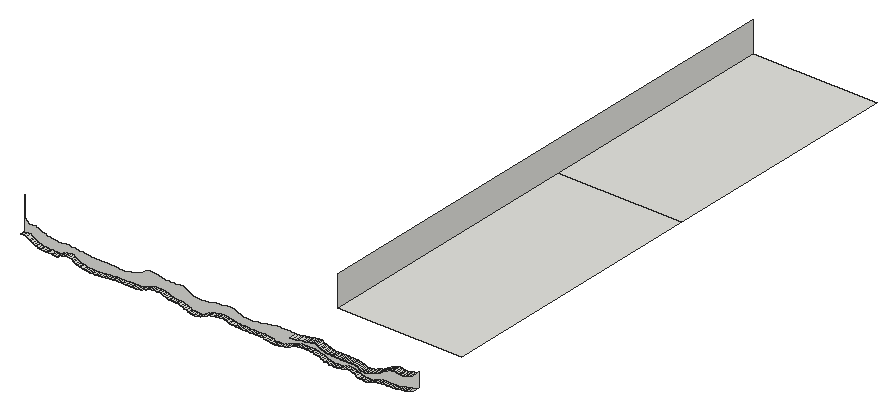
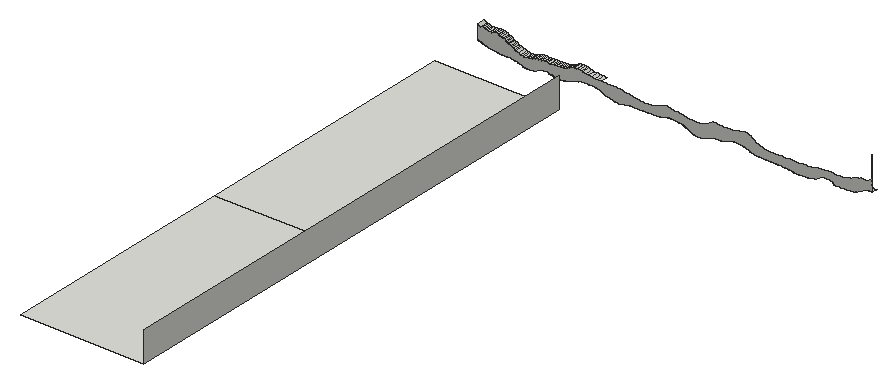
# SketchUp Ruby script. Lengths in inches.
U = 1.inch
M = Sketchup.active_model
def pt(a) = Geom::Point3d.new(a.map { |v| v * U })
def face(e, loops, mat)
  f = e.add_face(loops[0].map { |a| pt(a) })
  loops[1..].each { |l| e.add_face(l.map { |a| pt(a) }).erase! }
  f.material = f.back_material = mat if mat
  f
end
# faces: each face lists its corners as indices into pts; further lists are holes
def faces(e, pts, list, mat = nil) = list.each { |f| face(e, (f[0].is_a?(Array) ? f : [f]).map { |l| l.map { |i| pts[i] } }, mat) }
# xy, xz, yz: faces in a plane at the given z, y or x. An outline is a flat list of corners, or four numbers for a rectangle; further outlines are holes
def ring(l) = l.size == 4 ? [[l[0], l[1]], [l[2], l[1]], [l[2], l[3]], [l[0], l[3]]] : l.each_slice(2).to_a
def flat(e, list, mat, &to3) = list.each { |f| face(e, (f[0].is_a?(Array) ? f : [f]).map { |l| ring(l).map { |u, v| to3.(u, v) } }, mat) }
def xy(e, z, list, mat = nil) = flat(e, list, mat) { |x, y| [x, y, z] }
def xz(e, y, list, mat = nil) = flat(e, list, mat) { |x, z| [x, y, z] }
def yz(e, x, list, mat = nil) = flat(e, list, mat) { |y, z| [x, y, z] }
def lines(e, pts, list) = list.each { |a, b| e.add_line(pt(pts[a]), pt(pts[b])) }
# prism: a flat outline (further loops are holes) pulled along v
def prism(e, loops, v, mat = nil)
  f = face(e, loops, mat); d = Geom::Vector3d.new(v.map { |x| x * U })
  f.pushpull(f.normal.samedirection?(d) ? d.length : -d.length)
end
def box(e, o, s, mat = nil) = prism(e, [[o, [o[0] + s[0], o[1], o[2]], [o[0] + s[0], o[1] + s[1], o[2]], [o[0], o[1] + s[1], o[2]]]], [0, 0, s[2]], mat)
def at(x, y, z, deg = 0) = Geom::Transformation.translation(pt([x, y, z])) * Geom::Transformation.rotation(ORIGIN, Z_AXIS, deg.degrees)
def axes(o, x, y, z) = Geom::Transformation.new([*x, 0, *y, 0, *z, 0, *pt(o).to_a, 1])
def part(name) = M.definitions.add(name)
# library, detail: a bought-in or finely detailed component or shape, given as its bounding box
def library(name, o, s) = part(name).tap { |d| box(d.entities, o, s) }
def detail(e, o, s) = box(e.add_group.entities, o, s)
def put(e, d, t, mat = nil) = e.add_instance(d, t).tap { |i| i.material = mat if mat }
def group(e, t, mat = nil) = e.add_group.tap { |g| g.transformation = t; g.material = mat if mat }.entities
root = M.entities
xy(root,237.65,[[2039.58,2402.3,2040.27,2404.3],[2040.27,2402.3,2040.89,2404.3]])
xy(root,238.18,[[2133.53,2402.3,2134.21,2404.3]])
xy(root,238.33,[[2048.68,2402.3,2049.23,2404.3],[2049.23,2402.3,2049.91,2404.3]])
xy(root,238.34,[[2050.59,2402.3,2051.52,2404.3],[2051.52,2402.3,2052.01,2404.3],[2052.01,2402.3,2052.77,2404.3],[2052.77,2402.3,2053.4,2404.3],[2053.4,2402.3,2054.15,2404.3],
  [2054.15,2402.3,2054.77,2404.3],[2054.77,2402.3,2055.54,2404.3],[2055.54,2402.3,2056.16,2404.3]])
xy(root,238.62,[[2100.06,2402.3,2100.83,2404.3],[2100.83,2402.3,2101.46,2404.3],[2101.46,2402.3,2102.22,2404.3],[2102.22,2402.3,2102.84,2404.3],[2102.84,2402.3,2103.69,2404.3],
  [2103.69,2402.3,2104.33,2404.3],[2104.33,2402.3,2104.95,2404.3]])
xy(root,238.625,[[2098.64,2402.3,2099.5,2404.3]])
xy(root,238.89,[[2154.45,2402.3,2155.13,2404.3]])
xy(root,238.9,[[2155.89,2402.3,2156.51,2404.3],[2156.51,2402.3,2157.28,2404.3]])
xy(root,240.43,[[2122.73,2402.3,2123.3,2404.3]])
xy(root,241.52,[[2010.28,2402.3,2010.34,2404.3]])
xy(root,242.28,[[2140.55,2401.37,2141.0625,2404.3]])
xy(root,242.3,[[2138.79,2401.37,2139.46,2404.3]])
xy(root,242.33,[[2136.38,2401.37,2136.96,2404.3]])
xy(root,242.625,[[2115.89,2425.46,2164.35,2532.83],[2115.89,2532.83,2164.35,2628.15]])
xz(root,2404.3,[[2079.2,236.98,2078.59,237.01,2077.9,237.04,2077.14,237.11,2076.45,237.2,2075.92,237.33,2075.25,237.68,2074.3125,237.96,2073.75,238.28,2072.97,238.43,2072.19,238.78,2071.52,238.79,2070.98,238.8,2070.22,238.83,2069.47,238.875,2068.9,238.94,2068.32,239.04,2067.66,239.29,2067.08,239.53,2066.55,239.7,2065.86,239.92,2065.23,240.11,2064.45,240.27,2063.83,240.25,2063.125,240.23,2062.36,240.19,2061.6875,240.12,2061.03,240.03,2060.39,239.85,2059.84,239.52,2059.28,239.35,2058.69,239.18,2058.18,238.86,2057.49,238.72,2056.67,238.59,2056.16,238.34,2050.59,238.34,2049.91,238.33,2048.68,238.33,2047.96,238.32,2047.11,238.3,2046.48,238.28,2045.73,238.26,2045.1,238.15,2044.34,238.13,2043.79,238.1,2042.9375,237.98,2042.32,237.94,2041.56,237.89,2040.89,237.65,2039.58,237.65,2038.89,237.66,2038.14,237.67,2037.54,237.68,2036.93,237.71,2036.22,237.76,2035.53,237.82,2034.87,237.9,2033.93,238.21,2033.46,238.31,2032.55,238.43,2031.9,238.74,2031.32,239.11,2030.74,239.38,2030.28,239.71,2029.58,240.11,2028.89,240.09,2028.23,240.05,2027.64,239.99,2026.91,239.88,2026.36,239.69,2025.78,239.55,2025.22,238.9375,2024.69,238.77,2023.95,238.79,2023.08,238.8,2022.57,238.82,2021.53,238.92,2020.84,238.93,2020.14,238.94,2019.44,238.97,2018.76,239.03,2018.07,239.09,2017.29,239.19,2016.78,239.52,2016.22,239.64,2015.77,239.86,2014.98,240.2,2014.38,240.59,2013.84,240.85,2012.82,241.55,2011.55,241.69,2010.34,241.52,2010.34,246.2,2011.91,244.96,2013.3,244.9375,2014.55,244.92,2014.77,244.61,2015.33,244.54,2016.09,244.41,2016.76,244.11,2017.28,243.95,2017.94,243.79,2018.46,243.48,2019.1,243.3,2019.6875,243.14,2020.17,243.06,2020.89,242.85,2021.47,242.78,2022.28,242.73,2022.82,242.68,2023.49,242.51,2024.01,242.46,2024.55,242.58,2025.18,242.57,2025.81,242.81,2026.38,242.86,2026.94,242.89,2027.58,242.92,2028.01,242.625,2028.62,242.65,2029.17,242.62,2029.8,242.58,2030.36,242.57,2031,242.48,2031.66,242.38,2032.32,242.34,2032.99,242.24,2034.16,241.96,2034.93,241.89,2035.75,241.83,2036.35,241.78,2037.12,241.75,2037.57,241.74,2038.12,241.72,2039.38,241.7,2040.11,241.69,2040.78,241.68,2041.37,241.68,2041.86,241.67,2042.5625,241.74,2043.13,241.75,2045.13,241.75,2045.62,241.67,2046.15,241.66,2046.76,241.57,2047.3,241.53,2047.92,241.51,2048.47,241.49,2049.17,241.48,2049.83,241.47,2050.4,241.46,2051.11,241.6,2051.84,241.85,2052.51,241.91,2053.41,242.1,2054.18,242.46,2054.88,242.78,2055.65,242.97,2056.18,243.23,2056.58,243.48,2057.1,243.72,2057.4375,244.12,2057.91,244.39,2058.39,244.73,2058.875,244.87,2059.46,244.95,2060.14,245.01,2060.79,244.81,2061.36,244.7,2061.84,244.67,2062.45,244.55,2062.99,244.51,2063.45,244.25,2064.2,244.11,2064.76,244.04,2065.38,243.99,2066.1,243.95,2066.6,243.93,2067.29,243.91,2067.86,243.89,2068.56,243.88,2069.21,243.94,2069.85,243.95,2070.41,244.1,2071.04,244.13,2071.52,244.15,2072.04,244.17,2072.56,244.18,2073.16,243.8,2073.7,243.43,2074.31,243.09,2074.7,242.875,2075.2,242.68,2075.79,242.51,2076.3,242.21,2076.9,242.11,2077.58,241.96,2078.14,241.89,2078.6,241.85,2079.12,241.8125,2079.63,241.79,2080.21,241.78,2080.88,241.91,2081.35,241.93,2082.02,242.09,2082.79,242.2,2083.29,242.24,2083.9,242.42,2084.45,242.47,2085.2,242.71,2085.84,242.78,2086.32,242.82,2087.01,242.85,2087.71,242.87,2088.26,243.02,2088.88,243.05,2089.43,243.29,2090.11,243.35,2090.66,243.39,2091.26,243.42,2092.03,243.14,2092.6,242.9375,2093.15,242.65,2093.77,242.39,2094.53,242.14,2095.17,241.89,2095.66,241.78,2096.71,241.63,2097.48,241.56,2098.08,241.51,2098.53,241.48,2099.05,241.46,2099.92,241.51,2100.64,241.59,2101.58,241.82,2102.36,241.87,2103.125,241.98,2103.74,242.02,2104.39,242.19,2105.09,242.38,2105.58,242.4375,2106.1,242.48,2106.76,242.58,2107.29,242.61,2107.875,242.77,2108.33,242.95,2108.89,243.01,2109.4,243.05,2109.97,243.08,2110.625,243.09,2112.78,243.09,2113.35,243.08,2113.9375,243.07,2114.52,243.07,2115.18,243.0625,2115.79,243.05,2116.47,243.05,2117.74,243.1,2118.91,243.17,2120.05,243.4,2121.3125,243.52,2122.44,243.71,2123.34,243.99,2124.04,244.08,2124.74,244.21,2125.32,244.27,2125.86,244.3,2126.53,244.39,2127.125,244.19,2127.5,243.88,2127.98,243.59,2128.53,243.33,2129.08,243.22,2129.57,242.92,2130.05,242.75,2130.61,242.6,2131.17,242.52,2131.73,242.47,2132.3125,242.43,2132.89,242.4,2133.47,242.39,2134.05,242.37,2134.63,242.36,2135.22,242.35,2136.38,242.33,2136.96,242.33,2137.68,242.32,2138.15,242.3125,2138.79,242.3,2139.46,242.3,2139.91,242.29,2140.55,242.28,2141.0625,242.28,2141.69,242.2,2142.27,241.97,2142.84,241.84,2143.35,241.57,2143.77,241.33,2144.24,241.24,2144.77,241.17,2145.24,241.12,2145.84,241.09,2146.41,241.14,2147.05,241.35,2147.64,241.46,2148.58,241.85,2149.58,242.23,2150.14,242.42,2150.86,242.61,2151.375,242.91,2151.75,243.14,2152.29,243.52,2152.77,243.71,2153.1,244.02,2153.54,244.21,2154.13,244.57,2154.6,244.76,2155.22,245.125,2155.72,245.32,2156.2,245.41,2156.75,245.48,2157.24,245.59,2157.77,245.55,2158.38,245.35,2158.87,245.31,2159.42,245.27,2159.98,245.24,2160.54,245.22,2161.1,245.34,2161.73,245.42,2162.3125,245.52,2162.69,245.76,2163.16,245.9,2164.35,246.43,2164.35,240.89,2162.52,240.1,2161.96,239.96,2161.4375,239.81,2160.75,239.53,2160.2,239.49,2159.48,239.42,2158.68,239.28,2157.91,239.15,2157.28,238.9,2155.89,238.9,2155.13,238.89,2154.45,238.89,2153.77,238.88,2153.23,238.875,2152.47,238.86,2151.73,238.83,2151.16,238.8,2150.58,238.74,2149.92,238.6,2149.35,238.51,2148.82,238.33,2148.13,238.08,2147.45,237.84,2146.76,237.5625,2146.16,237.47,2145.48,237.4,2144.75,237.42,2144.18,237.45,2143.59,237.51,2142.99,237.59,2142.45,237.71,2141.62,238,2140.91,238.33,2140.36,238.57,2139.86,238.86,2139.34,238.96,2138.65,239.02,2137.97,239.125,2137.23,239.04,2136.66,238.66,2136.07,238.61,2135.41,238.55,2134.89,238.27,2134.21,238.18,2133.53,238.18,2132.86,238.11,2132.33,238.15,2131.51,238.19,2130.9375,238.26,2130.37,238.48,2129.71,238.56,2129.14,238.67,2128.62,239.01,2127.9375,239.18,2127.3125,239.5,2126.55,239.65,2125.9375,239.8,2125.18,239.96,2124.53,240.23,2123.95,240.27,2123.3,240.43,2122.73,240.43,2122.15,240.42,2121.625,240.41,2120.93,240.4,2120.24,240.37,2119.55,240.33,2118.87,240.27,2118.19,240.17,2117.57,239.97,2116.92,239.75,2116.18,239.375,2115.39,239.08,2114.51,238.72,2113.76,238.46,2112.54,238.14,2111.42,237.88,2110.77,237.87,2109.9,237.74,2109.19,237.79,2108.42,237.86,2107.79,238.15,2107.02,238.19,2106.4,238.25,2105.64,238.45,2104.95,238.62,2100.06,238.62,2099.5,238.625,2098.64,238.625,2097.95,238.63,2097.33,238.64,2096.55,238.65,2095.88,238.66,2095.19,238.6875,2094.52,238.73,2094.04,238.78,2093.16,238.93,2092.39,239.07,2091.84,239.16,2090.99,239.44,2090.32,239.56,2089.71,239.72,2088.98,239.7,2088.42,239.69,2087.83,239.65,2087.21,239.6,2086.72,239.54,2085.91,239.31,2084.91,239.22,2084.33,239.12,2083.6875,238.76,2083.05,238.51,2082.49,238.375,2082.05,238.02,2081.35,237.74,2080.73,237.43,2079.88,237.22],[2010.28,241.52,2010.34,254.5]])
yz(root,2115.89,[[2425.46,242.625,2628.15,254.5]])
p = [[2077.14,2404.3,237.11],[2077.9,2404.3,237.04],[2077.9,2402.3,237.04],[2077.14,2402.3,237.11],[2078.59,2404.3,237.01],[2078.59,2402.3,237.01],
  [2079.2,2404.3,236.98],[2079.2,2402.3,236.98],[2079.88,2404.3,237.22],[2079.88,2402.3,237.22],[2076.45,2404.3,237.2],[2076.45,2402.3,237.2],
  [2075.92,2404.3,237.33],[2075.92,2402.3,237.33],[2080.73,2404.3,237.43],[2080.73,2402.3,237.43],[2075.25,2404.3,237.68],[2075.25,2402.3,237.68],
  [2081.35,2404.3,237.74],[2081.35,2402.3,237.74],[2144.18,2404.3,237.45],[2144.75,2404.3,237.42],[2144.75,2402.3,237.42],[2144.18,2402.3,237.45],
  [2145.48,2404.3,237.4],[2145.48,2402.3,237.4],[2146.16,2404.3,237.47],[2146.16,2402.3,237.47],[2142.99,2404.3,237.59],[2143.59,2404.3,237.51],
  [2143.59,2402.3,237.51],[2142.99,2402.3,237.59],[2146.76,2404.3,237.5625],[2146.76,2402.3,237.5625],[2040.89,2404.3,237.65],[2041.56,2404.3,237.89],
  [2041.56,2402.3,237.89],[2040.89,2402.3,237.65],[2142.45,2404.3,237.71],[2142.45,2402.3,237.71],[2147.45,2404.3,237.84],[2147.45,2402.3,237.84],
  [2036.22,2404.3,237.76],[2036.93,2404.3,237.71],[2036.93,2402.3,237.71],[2036.22,2402.3,237.76],[2037.54,2404.3,237.68],[2037.54,2402.3,237.68],
  [2038.14,2404.3,237.67],[2038.14,2402.3,237.67],[2038.89,2404.3,237.66],[2038.89,2402.3,237.66],[2039.58,2404.3,237.65],[2039.58,2402.3,237.65],
  [2074.3125,2404.3,237.96],[2074.3125,2402.3,237.96],[2082.05,2404.3,238.02],[2082.05,2402.3,238.02],[2109.19,2404.3,237.79],[2109.9,2404.3,237.74],
  [2109.9,2402.3,237.74],[2109.19,2402.3,237.79],[2110.77,2404.3,237.87],[2110.77,2402.3,237.87],[2141.62,2404.3,238],[2141.62,2402.3,238],
  [2034.87,2404.3,237.9],[2035.53,2404.3,237.82],[2035.53,2402.3,237.82],[2034.87,2402.3,237.9],[2108.42,2404.3,237.86],[2108.42,2402.3,237.86],
  [2148.13,2404.3,238.08],[2148.13,2402.3,238.08],[2033.93,2404.3,238.21],[2033.93,2402.3,238.21],[2042.32,2404.3,237.94],[2042.32,2402.3,237.94],
  [2042.9375,2404.3,237.98],[2042.9375,2402.3,237.98],[2107.79,2404.3,238.15],[2107.79,2402.3,238.15],[2111.42,2404.3,237.88],[2111.42,2402.3,237.88],
  [2112.54,2404.3,238.14],[2112.54,2402.3,238.14],[2043.79,2404.3,238.1],[2043.79,2402.3,238.1],[2073.75,2404.3,238.28],[2073.75,2402.3,238.28],
  [2082.49,2404.3,238.375],[2082.49,2402.3,238.375],[2140.91,2404.3,238.33],[2140.91,2402.3,238.33],[2044.34,2404.3,238.13],[2044.34,2402.3,238.13],
  [2045.1,2404.3,238.15],[2045.1,2402.3,238.15],[2107.02,2404.3,238.19],[2107.02,2402.3,238.19],[2113.76,2404.3,238.46],[2113.76,2402.3,238.46],
  [2131.51,2404.3,238.19],[2132.33,2404.3,238.15],[2132.33,2402.3,238.15],[2131.51,2402.3,238.19],[2132.86,2404.3,238.11],[2132.86,2402.3,238.11],
  [2133.53,2404.3,238.18],[2133.53,2402.3,238.18],[2148.82,2404.3,238.33],[2148.82,2402.3,238.33],[2033.46,2404.3,238.31],[2033.46,2402.3,238.31],
  [2045.73,2404.3,238.26],[2045.73,2402.3,238.26],[2106.4,2404.3,238.25],[2106.4,2402.3,238.25],[2130.9375,2404.3,238.26],[2130.9375,2402.3,238.26],
  [2134.21,2404.3,238.18],[2134.89,2404.3,238.27],[2134.89,2402.3,238.27],[2134.21,2402.3,238.18],[2032.55,2404.3,238.43],[2032.55,2402.3,238.43],
  [2046.48,2404.3,238.28],[2046.48,2402.3,238.28],[2047.11,2404.3,238.3],[2047.11,2402.3,238.3],[2047.96,2404.3,238.32],[2047.96,2402.3,238.32],
  [2048.68,2404.3,238.33],[2048.68,2402.3,238.33],[2049.91,2404.3,238.33],[2050.59,2404.3,238.34],[2050.59,2402.3,238.34],[2049.91,2402.3,238.33],
  [2056.16,2404.3,238.34],[2056.67,2404.3,238.59],[2056.67,2402.3,238.59],[2056.16,2402.3,238.34],[2072.97,2404.3,238.43],[2072.97,2402.3,238.43],
  [2105.64,2404.3,238.45],[2105.64,2402.3,238.45],[2130.37,2404.3,238.48],[2130.37,2402.3,238.48],[2135.41,2404.3,238.55],[2135.41,2402.3,238.55],
  [2140.36,2404.3,238.57],[2140.36,2402.3,238.57],[2149.35,2404.3,238.51],[2149.35,2402.3,238.51],[2031.9,2404.3,238.74],[2031.9,2402.3,238.74],
  [2072.19,2404.3,238.78],[2072.19,2402.3,238.78],[2083.05,2404.3,238.51],[2083.05,2402.3,238.51],[2083.6875,2404.3,238.76],[2083.6875,2402.3,238.76],
  [2104.95,2404.3,238.62],[2104.95,2402.3,238.62],[2114.51,2404.3,238.72],[2114.51,2402.3,238.72],[2129.71,2404.3,238.56],[2129.71,2402.3,238.56],
  [2136.07,2404.3,238.61],[2136.07,2402.3,238.61],[2149.92,2404.3,238.6],[2149.92,2402.3,238.6],[2057.49,2404.3,238.72],[2057.49,2402.3,238.72],
  [2095.88,2404.3,238.66],[2096.55,2404.3,238.65],[2096.55,2402.3,238.65],[2095.88,2402.3,238.66],[2097.33,2404.3,238.64],[2097.33,2402.3,238.64],
  [2097.95,2404.3,238.63],[2097.95,2402.3,238.63],[2098.64,2404.3,238.625],[2098.64,2402.3,238.625],[2099.5,2404.3,238.625],[2100.06,2404.3,238.62],
  [2100.06,2402.3,238.62],[2099.5,2402.3,238.625],[2129.14,2404.3,238.67],[2129.14,2402.3,238.67],[2136.66,2404.3,238.66],[2136.66,2402.3,238.66],
  [2139.86,2404.3,238.86],[2139.86,2402.3,238.86],[2150.58,2404.3,238.74],[2150.58,2402.3,238.74],[2031.32,2404.3,239.11],[2031.32,2402.3,239.11],
  [2058.18,2404.3,238.86],[2058.18,2402.3,238.86],[2094.04,2404.3,238.78],[2094.52,2404.3,238.73],[2094.52,2402.3,238.73],[2094.04,2402.3,238.78],
  [2095.19,2404.3,238.6875],[2095.19,2402.3,238.6875],[2115.39,2404.3,239.08],[2115.39,2402.3,239.08],[2128.62,2404.3,239.01],[2128.62,2402.3,239.01],
  [2137.23,2404.3,239.04],[2137.23,2402.3,239.04],[2151.16,2404.3,238.8],[2151.16,2402.3,238.8],[2021.53,2404.3,238.92],[2022.57,2404.3,238.82],
  [2022.57,2402.3,238.82],[2021.53,2402.3,238.92],[2023.08,2404.3,238.8],[2023.08,2402.3,238.8],[2023.95,2404.3,238.79],[2023.95,2402.3,238.79],
  [2024.69,2404.3,238.77],[2024.69,2402.3,238.77],[2025.22,2404.3,238.9375],[2025.22,2402.3,238.9375],[2069.47,2404.3,238.875],[2070.22,2404.3,238.83],
  [2070.22,2402.3,238.83],[2069.47,2402.3,238.875],[2070.98,2404.3,238.8],[2070.98,2402.3,238.8],[2071.52,2404.3,238.79],[2071.52,2402.3,238.79],
  [2084.33,2404.3,239.12],[2084.33,2402.3,239.12],[2093.16,2404.3,238.93],[2093.16,2402.3,238.93],[2151.73,2404.3,238.83],[2151.73,2402.3,238.83],
  [2152.47,2404.3,238.86],[2152.47,2402.3,238.86],[2019.44,2404.3,238.97],[2020.14,2404.3,238.94],[2020.14,2402.3,238.94],[2019.44,2402.3,238.97],
  [2020.84,2404.3,238.93],[2020.84,2402.3,238.93],[2025.78,2404.3,239.55],[2025.78,2402.3,239.55],[2058.69,2404.3,239.18],[2058.69,2402.3,239.18],
  [2068.32,2404.3,239.04],[2068.9,2404.3,238.94],[2068.9,2402.3,238.94],[2068.32,2402.3,239.04],[2092.39,2404.3,239.07],[2092.39,2402.3,239.07],
  [2139.34,2404.3,238.96],[2139.34,2402.3,238.96],[2153.23,2404.3,238.875],[2153.23,2402.3,238.875],[2153.77,2404.3,238.88],[2153.77,2402.3,238.88],
  [2154.45,2404.3,238.89],[2154.45,2402.3,238.89],[2155.13,2404.3,238.89],[2155.89,2404.3,238.9],[2155.89,2402.3,238.9],[2155.13,2402.3,238.89],
  [2157.28,2404.3,238.9],[2157.91,2404.3,239.15],[2157.91,2402.3,239.15],[2157.28,2402.3,238.9],[2018.07,2404.3,239.09],[2018.76,2404.3,239.03],
  [2018.76,2402.3,239.03],[2018.07,2402.3,239.09],[2067.66,2404.3,239.29],[2067.66,2402.3,239.29],[2127.9375,2404.3,239.18],[2127.9375,2402.3,239.18],
  [2137.97,2404.3,239.125],[2137.97,2402.3,239.125],[2138.65,2404.3,239.02],[2138.65,2402.3,239.02],[2017.29,2404.3,239.19],[2017.29,2402.3,239.19],
  [2030.74,2404.3,239.38],[2030.74,2402.3,239.38],[2084.91,2404.3,239.22],[2084.91,2402.3,239.22],[2091.84,2404.3,239.16],[2091.84,2402.3,239.16],
  [2116.18,2404.3,239.375],[2116.18,2402.3,239.375],[2016.78,2404.3,239.52],[2016.78,2402.3,239.52],[2059.28,2404.3,239.35],[2059.28,2402.3,239.35],
  [2085.91,2404.3,239.31],[2085.91,2402.3,239.31],[2090.99,2404.3,239.44],[2090.99,2402.3,239.44],[2127.3125,2404.3,239.5],[2127.3125,2402.3,239.5],
  [2158.68,2404.3,239.28],[2158.68,2402.3,239.28],[2067.08,2404.3,239.53],[2067.08,2402.3,239.53],[2086.72,2404.3,239.54],[2086.72,2402.3,239.54],
  [2159.48,2404.3,239.42],[2159.48,2402.3,239.42],[2030.28,2404.3,239.71],[2030.28,2402.3,239.71],[2059.84,2404.3,239.52],[2059.84,2402.3,239.52],
  [2090.32,2404.3,239.56],[2090.32,2402.3,239.56],[2116.92,2404.3,239.75],[2116.92,2402.3,239.75],[2160.2,2404.3,239.49],[2160.2,2402.3,239.49],
  [2016.22,2404.3,239.64],[2016.22,2402.3,239.64],[2060.39,2404.3,239.85],[2060.39,2402.3,239.85],[2066.55,2404.3,239.7],[2066.55,2402.3,239.7],
  [2087.21,2404.3,239.6],[2087.21,2402.3,239.6],[2126.55,2404.3,239.65],[2126.55,2402.3,239.65],[2160.75,2404.3,239.53],[2160.75,2402.3,239.53],
  [2161.4375,2404.3,239.81],[2161.4375,2402.3,239.81],[2015.77,2404.3,239.86],[2015.77,2402.3,239.86],[2026.36,2404.3,239.69],[2026.36,2402.3,239.69],
  [2087.83,2404.3,239.65],[2087.83,2402.3,239.65],[2088.42,2404.3,239.69],[2088.42,2402.3,239.69],[2089.71,2404.3,239.72],[2089.71,2402.3,239.72],
  [2026.91,2404.3,239.88],[2026.91,2402.3,239.88],[2029.58,2404.3,240.11],[2029.58,2402.3,240.11],[2065.86,2404.3,239.92],[2065.86,2402.3,239.92],
  [2088.98,2404.3,239.7],[2088.98,2402.3,239.7],[2117.57,2404.3,239.97],[2117.57,2402.3,239.97],[2125.9375,2404.3,239.8],[2125.9375,2402.3,239.8],
  [2061.03,2404.3,240.03],[2061.03,2402.3,240.03],[2125.18,2404.3,239.96],[2125.18,2402.3,239.96],[2161.96,2404.3,239.96],[2161.96,2402.3,239.96],
  [2014.98,2404.3,240.2],[2014.98,2402.3,240.2],[2027.64,2404.3,239.99],[2027.64,2402.3,239.99],[2065.23,2404.3,240.11],[2065.23,2402.3,240.11],
  [2028.23,2404.3,240.05],[2028.23,2402.3,240.05],[2028.89,2404.3,240.09],[2028.89,2402.3,240.09],[2061.6875,2404.3,240.12],[2061.6875,2402.3,240.12],
  [2118.19,2404.3,240.17],[2118.19,2402.3,240.17],[2124.53,2404.3,240.23],[2124.53,2402.3,240.23],[2162.52,2404.3,240.1],[2162.52,2402.3,240.1],
  [2062.36,2404.3,240.19],[2062.36,2402.3,240.19],[2064.45,2404.3,240.27],[2064.45,2402.3,240.27],[2164.35,2404.3,240.89],[2164.35,2402.3,240.89],
  [2014.38,2404.3,240.59],[2014.38,2402.3,240.59],[2063.125,2404.3,240.23],[2063.125,2402.3,240.23],[2063.83,2404.3,240.25],[2063.83,2402.3,240.25],
  [2118.87,2404.3,240.27],[2118.87,2402.3,240.27],[2123.95,2404.3,240.27],[2123.95,2402.3,240.27],[2119.55,2404.3,240.33],[2119.55,2402.3,240.33],
  [2120.24,2404.3,240.37],[2120.24,2402.3,240.37],[2123.3,2404.3,240.43],[2123.3,2402.3,240.43],[2120.93,2404.3,240.4],[2120.93,2402.3,240.4],
  [2121.625,2404.3,240.41],[2121.625,2402.3,240.41],[2122.15,2404.3,240.42],[2122.15,2402.3,240.42],[2122.73,2404.3,240.43],[2122.73,2402.3,240.43],
  [2013.84,2404.3,240.85],[2013.84,2402.3,240.85],[2012.82,2404.3,241.55],[2012.82,2402.3,241.55],[2144.77,2404.3,241.17],[2145.24,2404.3,241.12],
  [2145.24,2401.37,241.12],[2144.77,2401.37,241.17],[2145.84,2404.3,241.09],[2145.84,2401.37,241.09],[2146.41,2404.3,241.14],[2146.41,2401.37,241.14],
  [2147.05,2404.3,241.35],[2147.05,2401.37,241.35],[2143.77,2404.3,241.33],[2144.24,2404.3,241.24],[2144.24,2401.37,241.24],[2143.77,2401.37,241.33],
  [2143.35,2404.3,241.57],[2143.35,2401.37,241.57],[2147.64,2404.3,241.46],[2147.64,2401.37,241.46],[2148.58,2404.3,241.85],[2148.58,2401.37,241.85],
  [2010.34,2404.3,241.52],[2011.55,2404.3,241.69],[2011.55,2402.3,241.69],[2010.34,2402.3,241.52],[2142.84,2404.3,241.84],[2142.84,2401.37,241.84],
  [2142.27,2404.3,241.97],[2142.27,2401.37,241.97],[2149.58,2404.3,242.23],[2149.58,2401.37,242.23],[2141.69,2404.3,242.2],[2141.69,2401.37,242.2],
  [2141.0625,2404.3,242.28],[2141.0625,2401.37,242.28],[2150.14,2404.3,242.42],[2150.14,2401.37,242.42],[2135.22,2404.3,242.35],[2135.8,2404.3,242.34],
  [2135.8,2401.37,242.34],[2135.22,2401.37,242.35],[2136.38,2404.3,242.33],[2136.38,2401.37,242.33],[2136.96,2404.3,242.33],[2137.68,2404.3,242.32],
  [2137.68,2401.37,242.32],[2136.96,2401.37,242.33],[2138.15,2404.3,242.3125],[2138.15,2401.37,242.3125],[2138.79,2404.3,242.3],[2138.79,2401.37,242.3],
  [2139.46,2404.3,242.3],[2139.91,2404.3,242.29],[2139.91,2401.37,242.29],[2139.46,2401.37,242.3],[2140.55,2404.3,242.28],[2140.55,2401.37,242.28],
  [2131.73,2404.3,242.47],[2132.3125,2404.3,242.43],[2132.3125,2401.37,242.43],[2131.73,2401.37,242.47],[2132.89,2404.3,242.4],[2132.89,2401.37,242.4],
  [2133.47,2404.3,242.39],[2133.47,2401.37,242.39],[2134.05,2404.3,242.37],[2134.05,2401.37,242.37],[2134.63,2404.3,242.36],[2134.63,2401.37,242.36],
  [2150.86,2404.3,242.61],[2150.86,2401.37,242.61],[2130.61,2404.3,242.6],[2131.17,2404.3,242.52],[2131.17,2401.37,242.52],[2130.61,2401.37,242.6],
  [2130.05,2404.3,242.75],[2130.05,2401.37,242.75],[2151.375,2404.3,242.91],[2151.375,2401.37,242.91],[2129.57,2404.3,242.92],[2129.57,2401.37,242.92],
  [2129.08,2404.3,243.22],[2129.08,2401.37,243.22],[2151.75,2404.3,243.14],[2151.75,2401.37,243.14],[2116.47,2404.3,243.05],[2117.74,2404.3,243.1],
  [2117.74,2401.37,243.1],[2116.47,2401.37,243.05],[2118.91,2404.3,243.17],[2118.91,2401.37,243.17],[2152.29,2404.3,243.52],[2152.29,2401.37,243.52],
  [2120.05,2404.3,243.4],[2120.05,2401.37,243.4],[2128.53,2404.3,243.33],[2128.53,2401.37,243.33],[2127.98,2404.3,243.59],[2127.98,2401.37,243.59],
  [2121.3125,2404.3,243.52],[2121.3125,2401.37,243.52],[2122.44,2404.3,243.71],[2122.44,2401.37,243.71],[2152.77,2404.3,243.71],[2152.77,2401.37,243.71],
  [2127.5,2404.3,243.88],[2127.5,2401.37,243.88],[2123.34,2404.3,243.99],[2123.34,2401.37,243.99],[2153.1,2404.3,244.02],[2153.1,2401.37,244.02],
  [2127.125,2404.3,244.19],[2127.125,2401.37,244.19],[2124.04,2404.3,244.08],[2124.04,2401.37,244.08],[2153.54,2404.3,244.21],[2153.54,2401.37,244.21],
  [2124.74,2404.3,244.21],[2124.74,2401.37,244.21],[2125.32,2404.3,244.27],[2125.32,2401.37,244.27],[2126.53,2404.3,244.39],[2126.53,2401.37,244.39],
  [2154.13,2404.3,244.57],[2154.13,2401.37,244.57],[2125.86,2404.3,244.3],[2125.86,2401.37,244.3],[2154.6,2404.3,244.76],[2154.6,2401.37,244.76],
  [2155.22,2404.3,245.125],[2155.22,2401.37,245.125],[2155.72,2404.3,245.32],[2155.72,2401.37,245.32],[2159.42,2404.3,245.27],[2159.98,2404.3,245.24],
  [2159.98,2401.37,245.24],[2159.42,2401.37,245.27],[2160.54,2404.3,245.22],[2160.54,2401.37,245.22],[2161.1,2404.3,245.34],[2161.1,2401.37,245.34],
  [2156.2,2404.3,245.41],[2156.2,2401.37,245.41],[2157.77,2404.3,245.55],[2158.38,2404.3,245.35],[2158.38,2401.37,245.35],[2157.77,2401.37,245.55],
  [2158.87,2404.3,245.31],[2158.87,2401.37,245.31],[2161.73,2404.3,245.42],[2161.73,2401.37,245.42],[2156.75,2404.3,245.48],[2156.75,2401.37,245.48],
  [2162.3125,2404.3,245.52],[2162.3125,2401.37,245.52],[2157.24,2404.3,245.59],[2157.24,2401.37,245.59],[2162.69,2404.3,245.76],[2162.69,2401.37,245.76],
  [2163.16,2404.3,245.9],[2163.16,2401.37,245.9],[2164.35,2404.3,246.43],[2164.35,2401.37,246.43]]
faces(root,p,[[0,1,2,3],[1,4,5,2],[4,6,7,5],[6,8,9,7],[10,0,3,11],[12,10,11,13],[8,14,15,9],[16,12,13,17],
  [14,18,19,15],[20,21,22,23],[21,24,25,22],[24,26,27,25],[28,29,30,31],[29,20,23,30],[26,32,33,27],[34,35,36,37],
  [38,28,31,39],[32,40,41,33],[42,43,44,45],[43,46,47,44],[46,48,49,47],[48,50,51,49],[50,52,53,51],[54,16,17,55],
  [18,56,57,19],[58,59,60,61],[59,62,63,60],[64,38,39,65],[66,67,68,69],[67,42,45,68],[70,58,61,71],[40,72,73,41],
  [74,66,69,75],[35,76,77,36],[76,78,79,77],[80,70,71,81],[62,82,83,63],[82,84,85,83],[78,86,87,79],[88,54,55,89],
  [56,90,91,57],[92,64,65,93],[86,94,95,87],[94,96,97,95],[98,80,81,99],[84,100,101,85],[102,103,104,105],[103,106,107,104],
  [106,108,109,107],[72,110,111,73],[112,74,75,113],[96,114,115,97],[116,98,99,117],[118,102,105,119],[120,121,122,123],[124,112,113,125],
  [114,126,127,115],[126,128,129,127],[128,130,131,129],[130,132,133,131],[134,135,136,137],[138,139,140,141],[142,88,89,143],[144,116,117,145],
  [146,118,119,147],[121,148,149,122],[150,92,93,151],[110,152,153,111],[154,124,125,155],[156,142,143,157],[90,158,159,91],[158,160,161,159],
  [162,144,145,163],[100,164,165,101],[166,146,147,167],[148,168,169,149],[152,170,171,153],[139,172,173,140],[174,175,176,177],[175,178,179,176],
  [178,180,181,179],[180,182,183,181],[184,185,186,187],[188,166,167,189],[168,190,191,169],[192,150,151,193],[170,194,195,171],[196,154,155,197],
  [172,198,199,173],[200,201,202,203],[201,204,205,202],[204,174,177,205],[164,206,207,165],[208,188,189,209],[190,210,211,191],[194,212,213,195],
  [214,215,216,217],[215,218,219,216],[218,220,221,219],[220,222,223,221],[222,224,225,223],[226,227,228,229],[227,230,231,228],[230,232,233,231],
  [232,156,157,233],[160,234,235,161],[236,200,203,237],[212,238,239,213],[238,240,241,239],[242,243,244,245],[243,246,247,244],[246,214,217,247],
  [224,248,249,225],[198,250,251,199],[252,253,254,255],[253,226,229,254],[256,236,237,257],[258,192,193,259],[240,260,261,241],[260,262,263,261],
  [262,264,265,263],[266,267,268,269],[270,271,272,273],[274,275,276,277],[275,242,245,276],[278,252,255,279],[280,208,209,281],[210,282,283,211],
  [282,284,285,283],[284,258,259,285],[286,274,277,287],[288,196,197,289],[234,290,291,235],[292,256,257,293],[206,294,295,207],[296,286,287,297],
  [250,298,299,251],[290,300,301,291],[302,292,293,303],[304,280,281,305],[271,306,307,272],[308,278,279,309],[300,310,311,301],[306,312,313,307],
  [314,288,289,315],[298,316,317,299],[318,302,303,319],[294,320,321,295],[312,322,323,313],[324,296,297,325],[316,326,327,317],[328,308,309,329],
  [310,330,331,311],[332,304,305,333],[322,334,335,323],[334,336,337,335],[338,324,325,339],[248,340,341,249],[330,342,343,331],[342,344,345,343],
  [346,318,319,347],[340,348,349,341],[350,314,315,351],[352,328,329,353],[344,354,355,345],[354,346,347,355],[320,356,357,321],[358,332,333,359],
  [326,360,361,327],[362,358,359,363],[336,364,365,337],[366,338,339,367],[348,368,369,349],[370,352,353,371],[368,372,373,369],[372,374,375,373],
  [360,376,377,361],[356,378,379,357],[380,362,363,381],[364,382,383,365],[374,350,351,375],[376,384,385,377],[386,370,371,387],[382,388,389,383],
  [390,366,367,391],[384,392,393,385],[392,394,395,393],[378,396,397,379],[398,380,381,399],[394,386,387,395],[396,400,401,397],[400,402,403,401],
  [404,398,399,405],[402,406,407,403],[406,408,409,407],[408,410,411,409],[410,412,413,411],[414,390,391,415],[416,414,415,417],[418,419,420,421],
  [419,422,423,420],[422,424,425,423],[424,426,427,425],[428,429,430,431],[429,418,421,430],[432,428,431,433],[426,434,435,427],[434,436,437,435],
  [438,439,440,441],[442,432,433,443],[439,416,417,440],[444,442,443,445],[436,446,447,437],[448,444,445,449],[450,448,449,451],[446,452,453,447],
  [454,455,456,457],[455,458,459,456],[460,461,462,463],[461,464,465,462],[464,466,467,465],[468,469,470,471],[469,472,473,470],[474,475,476,477],
  [475,478,479,476],[478,480,481,479],[480,482,483,481],[482,484,485,483],[484,454,457,485],[452,486,487,453],[488,489,490,491],[489,474,477,490],
  [492,488,491,493],[486,494,495,487],[496,492,493,497],[498,496,497,499],[494,500,501,495],[502,503,504,505],[503,506,507,504],[500,508,509,501],
  [506,510,511,507],[512,498,499,513],[514,512,513,515],[510,516,517,511],[516,518,519,517],[508,520,521,509],[522,514,515,523],[518,524,525,519],
  [520,526,527,521],[528,522,523,529],[524,530,531,525],[526,532,533,527],[530,534,535,531],[534,536,537,535],[538,528,529,539],[532,540,541,533],
  [536,542,543,537],[542,538,539,543],[540,544,545,541],[544,546,547,545],[546,548,549,547],[550,551,552,553],[551,554,555,552],[554,556,557,555],
  [548,558,559,549],[560,561,562,563],[561,564,565,562],[564,550,553,565],[556,566,567,557],[558,568,569,559],[566,570,571,567],[568,572,573,569],
  [570,574,575,571],[572,560,563,573],[574,576,577,575],[576,578,579,577]])
